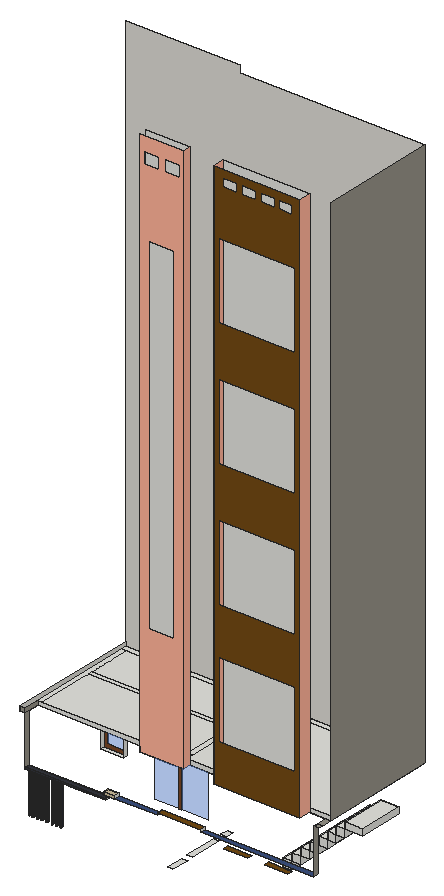
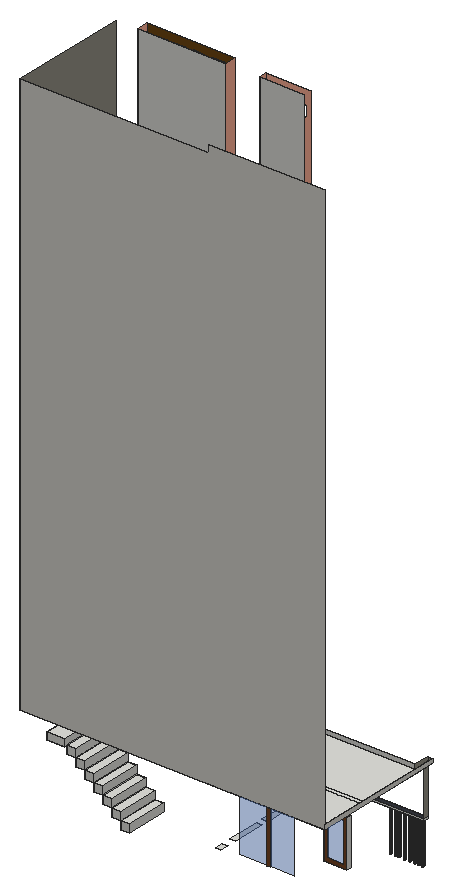
# SketchUp Ruby script. Lengths in inches.
U = 1.inch
M = Sketchup.active_model
def pt(a) = Geom::Point3d.new(a.map { |v| v * U })
def face(e, loops, mat)
  f = e.add_face(loops[0].map { |a| pt(a) })
  loops[1..].each { |l| e.add_face(l.map { |a| pt(a) }).erase! }
  f.material = f.back_material = mat if mat
  f
end
# faces: each face lists its corners as indices into pts; further lists are holes
def faces(e, pts, list, mat = nil) = list.each { |f| face(e, (f[0].is_a?(Array) ? f : [f]).map { |l| l.map { |i| pts[i] } }, mat) }
# xy, xz, yz: faces in a plane at the given z, y or x. An outline is a flat list of corners, or four numbers for a rectangle; further outlines are holes
def ring(l) = l.size == 4 ? [[l[0], l[1]], [l[2], l[1]], [l[2], l[3]], [l[0], l[3]]] : l.each_slice(2).to_a
def flat(e, list, mat, &to3) = list.each { |f| face(e, (f[0].is_a?(Array) ? f : [f]).map { |l| ring(l).map { |u, v| to3.(u, v) } }, mat) }
def xy(e, z, list, mat = nil) = flat(e, list, mat) { |x, y| [x, y, z] }
def xz(e, y, list, mat = nil) = flat(e, list, mat) { |x, z| [x, y, z] }
def yz(e, x, list, mat = nil) = flat(e, list, mat) { |y, z| [x, y, z] }
def lines(e, pts, list) = list.each { |a, b| e.add_line(pt(pts[a]), pt(pts[b])) }
# prism: a flat outline (further loops are holes) pulled along v
def prism(e, loops, v, mat = nil)
  f = face(e, loops, mat); d = Geom::Vector3d.new(v.map { |x| x * U })
  f.pushpull(f.normal.samedirection?(d) ? d.length : -d.length)
end
def box(e, o, s, mat = nil) = prism(e, [[o, [o[0] + s[0], o[1], o[2]], [o[0] + s[0], o[1] + s[1], o[2]], [o[0], o[1] + s[1], o[2]]]], [0, 0, s[2]], mat)
def at(x, y, z, deg = 0) = Geom::Transformation.translation(pt([x, y, z])) * Geom::Transformation.rotation(ORIGIN, Z_AXIS, deg.degrees)
def axes(o, x, y, z) = Geom::Transformation.new([*x, 0, *y, 0, *z, 0, *pt(o).to_a, 1])
def part(name) = M.definitions.add(name)
# library, detail: a bought-in or finely detailed component or shape, given as its bounding box
def library(name, o, s) = part(name).tap { |d| box(d.entities, o, s) }
def detail(e, o, s) = box(e.add_group.entities, o, s)
def put(e, d, t, mat = nil) = e.add_instance(d, t).tap { |i| i.material = mat if mat }
def group(e, t, mat = nil) = e.add_group.tap { |g| g.transformation = t; g.material = mat if mat }.entities
root = M.entities
M.materials.add("[Blinds Weave]").color = [114, 74, 20]
M.materials.add("[Color B02]").color = [255, 178, 153]
M.materials.add("[Formica Blue]").color = [58, 79, 124]
M.materials.add("[Formica Graystone]").color = [149, 146, 135]
M.materials.add("[Formica Laminate Dark]").color = [50, 53, 60]
M.materials.add("[Quartz Light Brown]").color = [199, 184, 152]
M.materials.add("[Terrazzo Tile Light]").color = [219, 217, 210]
M.materials.add("[Translucent Glass Blue]").color = [100, 149, 237]
M.materials["[Translucent Glass Blue]"].alpha = 0.5
M.materials.add("[Wood Veneer 01]").color = [120, 70, 37]
xy(root,9,[[405.97,32.04,421.1,82.09],[405.97,100.35,421.1,192.875],[405.97,220.7,421.1,243]])
xy(root,9.5,[[43.24,22.63,42.52,22.73,41.86,23,41.29,23.4375,40.85,24.01,40.58,24.67,40.49,25.38,40.58,26.09,40.85,26.76,41.29,27.33,41.86,27.76,42.52,28.04,43.24,28.13,43.95,28.04,44.61,27.76,45.18,27.33,45.62,26.76,45.89,26.09,45.99,25.38,45.89,24.67,45.62,24.01,45.18,23.4375,44.61,23,43.95,22.73]])
xy(root,90.32,[[48.09,243,111.9,254.6875]])
xy(root,121.625,[[575.75,18.26,642.4375,31.76],[690.75,18.26,757.4375,31.45]],"[Blinds Weave]")
xy(root,126.29,[[[13.78,18.26,120.72,32.04],[109.61,22.63,110.32,22.73,110.99,23,111.56,23.4375,111.99,24.01,112.27,24.67,112.36,25.38,112.27,26.09,111.99,26.76,111.56,27.33,110.99,27.76,110.32,28.04,109.61,28.13,108.9,28.04,108.24,27.76,107.67,27.33,107.23,26.76,106.95,26.09,106.86,25.38,106.95,24.67,107.23,24.01,107.67,23.4375,108.24,23,108.9,22.73],[96.86,22.63,97.57,22.73,98.24,23,98.81,23.4375,99.24,24.01,99.52,24.67,99.61,25.38,99.52,26.09,99.24,26.76,98.81,27.33,98.24,27.76,97.57,28.04,96.86,28.13,96.15,28.04,95.49,27.76,94.92,27.33,94.48,26.76,94.2,26.09,94.11,25.38,94.2,24.67,94.48,24.01,94.92,23.4375,95.49,23,96.15,22.73],[86.17,22.63,86.89,22.73,87.55,23,88.12,23.4375,88.55,24.01,88.83,24.67,88.92,25.38,88.83,26.09,88.55,26.76,88.12,27.33,87.55,27.76,86.89,28.04,86.17,28.13,85.46,28.04,84.8,27.76,84.23,27.33,83.79,26.76,83.52,26.09,83.42,25.38,83.52,24.67,83.79,24.01,84.23,23.4375,84.8,23,85.46,22.73],[70.8,22.63,71.51,22.73,72.17,23,72.74,23.4375,73.18,24.01,73.45,24.67,73.55,25.38,73.45,26.09,73.18,26.76,72.74,27.33,72.17,27.76,71.51,28.04,70.8,28.13,70.09,28.04,69.42,27.76,68.85,27.33,68.42,26.76,68.14,26.09,68.05,25.38,68.14,24.67,68.42,24.01,68.85,23.4375,69.42,23,70.09,22.73],[56.49,22.63,57.2,22.73,57.86,23,58.43,23.4375,58.87,24.01,59.14,24.67,59.24,25.38,59.14,26.09,58.87,26.76,58.43,27.33,57.86,27.76,57.2,28.04,56.49,28.13,55.77,28.04,55.11,27.76,54.54,27.33,54.1,26.76,53.83,26.09,53.74,25.38,53.83,24.67,54.1,24.01,54.54,23.4375,55.11,23,55.77,22.73],[43.24,22.63,43.95,22.73,44.61,23,45.18,23.4375,45.62,24.01,45.89,24.67,45.99,25.38,45.89,26.09,45.62,26.76,45.18,27.33,44.61,27.76,43.95,28.04,43.24,28.13,42.52,28.04,41.86,27.76,41.29,27.33,40.85,26.76,40.58,26.09,40.49,25.38,40.58,24.67,40.85,24.01,41.29,23.4375,41.86,23,42.52,22.73],[31.74,22.63,32.45,22.73,33.11,23,33.68,23.4375,34.12,24.01,34.39,24.67,34.49,25.38,34.39,26.09,34.12,26.76,33.68,27.33,33.11,27.76,32.45,28.04,31.74,28.13,31.02,28.04,30.36,27.76,29.79,27.33,29.35,26.76,29.08,26.09,28.99,25.38,29.08,24.67,29.35,24.01,29.79,23.4375,30.36,23,31.02,22.73],[20.55,22.63,21.26,22.73,21.92,23,22.49,23.4375,22.93,24.01,23.2,24.67,23.3,25.38,23.2,26.09,22.93,26.76,22.49,27.33,21.92,27.76,21.26,28.04,20.55,28.13,19.84,28.04,19.17,27.76,18.6,27.33,18.17,26.76,17.89,26.09,17.8,25.38,17.89,24.67,18.17,24.01,18.6,23.4375,19.17,23,19.84,22.73]],[131.16,18.26,141.6,32.04],[[141.6,18.26,240.76,32.04],[229.92,22.63,230.64,22.73,231.3,23,231.87,23.4375,232.3,24.01,232.58,24.67,232.67,25.38,232.58,26.09,232.3,26.76,231.87,27.33,231.3,27.76,230.64,28.04,229.92,28.13,229.21,28.04,228.55,27.76,227.98,27.33,227.54,26.76,227.27,26.09,227.17,25.38,227.27,24.67,227.54,24.01,227.98,23.4375,228.55,23,229.21,22.73],[218.67,22.63,219.39,22.73,220.05,23,220.62,23.4375,221.05,24.01,221.33,24.67,221.42,25.38,221.33,26.09,221.05,26.76,220.62,27.33,220.05,27.76,219.39,28.04,218.67,28.13,217.96,28.04,217.3,27.76,216.73,27.33,216.29,26.76,216.02,26.09,215.92,25.38,216.02,24.67,216.29,24.01,216.73,23.4375,217.3,23,217.96,22.73],[209.17,22.63,209.89,22.73,210.55,23,211.12,23.4375,211.55,24.01,211.83,24.67,211.92,25.38,211.83,26.09,211.55,26.76,211.12,27.33,210.55,27.76,209.89,28.04,209.17,28.13,208.46,28.04,207.8,27.76,207.23,27.33,206.79,26.76,206.52,26.09,206.42,25.38,206.52,24.67,206.79,24.01,207.23,23.4375,207.8,23,208.46,22.73],[197.05,22.63,197.76,22.73,198.42,23,198.99,23.4375,199.43,24.01,199.7,24.67,199.8,25.38,199.7,26.09,199.43,26.76,198.99,27.33,198.42,27.76,197.76,28.04,197.05,28.13,196.34,28.04,195.67,27.76,195.1,27.33,194.67,26.76,194.39,26.09,194.3,25.38,194.39,24.67,194.67,24.01,195.1,23.4375,195.67,23,196.34,22.73],[183.8,22.63,184.51,22.73,185.17,23,185.74,23.4375,186.18,24.01,186.45,24.67,186.55,25.38,186.45,26.09,186.18,26.76,185.74,27.33,185.17,27.76,184.51,28.04,183.8,28.13,183.09,28.04,182.42,27.76,181.85,27.33,181.42,26.76,181.14,26.09,181.05,25.38,181.14,24.67,181.42,24.01,181.85,23.4375,182.42,23,183.09,22.73],[171.74,22.63,172.45,22.73,173.11,23,173.68,23.4375,174.12,24.01,174.39,24.67,174.49,25.38,174.39,26.09,174.12,26.76,173.68,27.33,173.11,27.76,172.45,28.04,171.74,28.13,171.02,28.04,170.36,27.76,169.79,27.33,169.35,26.76,169.08,26.09,168.99,25.38,169.08,24.67,169.35,24.01,169.79,23.4375,170.36,23,171.02,22.73],[160.92,22.63,161.64,22.73,162.3,23,162.87,23.4375,163.3,24.01,163.58,24.67,163.67,25.38,163.58,26.09,163.3,26.76,162.87,27.33,162.3,27.76,161.64,28.04,160.92,28.13,160.21,28.04,159.55,27.76,158.98,27.33,158.54,26.76,158.27,26.09,158.17,25.38,158.27,24.67,158.54,24.01,158.98,23.4375,159.55,23,160.21,22.73],[150.24,22.63,150.95,22.73,151.61,23,152.18,23.4375,152.62,24.01,152.89,24.67,152.99,25.38,152.89,26.09,152.62,26.76,152.18,27.33,151.61,27.76,150.95,28.04,150.24,28.13,149.52,28.04,148.86,27.76,148.29,27.33,147.85,26.76,147.58,26.09,147.49,25.38,147.58,24.67,147.85,24.01,148.29,23.4375,148.86,23,149.52,22.73]]])
xy(root,130.36,[[13.78,18.26,240.76,32.04]],"[Formica Laminate Dark]")
xy(root,140.3125,[[237.58,15.64,265.93,18.26],[265.93,15.64,268.05,18.26],[237.58,18.26,240.76,32.04],[240.76,18.26,265.93,32.04],[265.93,18.26,268.05,32.04]])
xy(root,140.3125,[[268.05,18.26,388.35,32.04],[510.77,18.26,829.54,32.04]],"[Formica Blue]")
xy(root,146.9375,[[388.35,18.26,510.77,32.04]],"[Blinds Weave]")
xy(root,147.25,[[237.58,15.64,268.05,32.04]],"[Quartz Light Brown]")
xy(root,219.95,[[48.09,243,111.9,254.6875]])
xy(root,267.75,[[0,18.26,13.78,32.04],[538.37,28.0625,782.27,61.625],[0,32.04,13.78,377.76],[320.63,40.625,405.97,61.625],[405.97,40.625,421.1,61.625],
  [421.1,40.625,443.82,61.625],[13.78,61.625,405.97,243],[405.97,61.625,421.1,82.09],[421.1,61.625,829.54,377.76],[829.54,61.625,843.32,377.76],
  [405.97,82.09,421.1,100.35],[405.97,100.35,421.1,192.875],[405.97,192.875,421.1,220.7],[405.97,220.7,421.1,243],[13.78,243,405.97,255.17],
  [405.97,243,421.1,391.54],[13.78,255.17,405.97,377.76],[0,377.76,405.97,391.54],[421.1,377.76,843.32,391.54]])
xy(root,267.75,[[829.54,18.26,843.32,32.04],[829.54,32.04,843.32,61.625]],"[Formica Graystone]")
xz(root,15.64,[[237.58,140.3125,268.05,147.25]],"[Quartz Light Brown]")
xz(root,18.26,[[0,267.75,13.78,279.75]],"[Formica Graystone]")
xz(root,18.26,[[13.78,126.29,240.76,130.36]],"[Formica Laminate Dark]")
xz(root,28.0625,[[[538.37,267.75,782.27,1831.875],[552.31,378.36,767.87,593.92],[552.31,726.11,767.87,941.67],[552.31,1082.8,767.87,1298.36],[552.31,1440.48,767.87,1656.05],[565.47,1787.53,604,1811.34],[721.9,1787.53,760.43,1811.34],[618.59,1787.53,657.12,1811.34],[671.78,1787.53,710.31,1811.34]]],"[Blinds Weave]")
xz(root,32.04,[[13.78,126.29,240.76,130.36],[237.58,140.3125,268.05,147.25]])
xz(root,40.625,[[[320.63,267.75,443.82,1831.875],[345.55,586.3125,414.87,1568.875],[331.73,1759.52,372.85,1792.7],[390.85,1759.52,431.98,1792.7]]],"[Color B02]")
xz(root,61.625,[[13.78,267.75,320.63,279.75],[320.63,267.75,443.82,1831.875],[443.82,267.75,538.37,280.75],[538.37,267.75,782.27,1831.875],[782.27,267.75,843.32,278.91]])
xz(root,243,[[200.58,15.66,268.66,218.84],[278.13,15.66,352.51,218.84]],"[Translucent Glass Blue]")
xz(root,243,[[268.66,15.66,278.13,218.84]],"[Wood Veneer 01]")
xz(root,254.6875,[[57.74,99.98,102.25,210.29]],"[Translucent Glass Blue]")
xz(root,254.6875,[[[48.09,90.32,111.9,219.95],[57.74,99.98,102.25,210.29]]],"[Wood Veneer 01]")
xz(root,391.54,[[0,267.75,0,1852.125,320.63,1852.125,320.63,1831.875,843.32,1831.875,843.32,267.75]],"[Terrazzo Tile Light]")
yz(root,0,[[18.26,267.75,391.54,279.75]],"[Terrazzo Tile Light]")
yz(root,13.78,[[18.26,126.29,32.04,130.36]])
yz(root,13.78,[[18.26,130.36,32.04,267.75],[18.26,267.75,61.625,279.75]],"[Formica Graystone]")
yz(root,48.09,[[243,90.32,254.6875,219.95]])
yz(root,111.9,[[243,90.32,254.6875,219.95]])
yz(root,237.58,[[15.64,140.3125,32.04,147.25]],"[Quartz Light Brown]")
yz(root,240.76,[[18.26,126.29,32.04,130.36]])
yz(root,240.76,[[18.26,130.36,32.04,140.3125]],"[Quartz Light Brown]")
yz(root,268.05,[[15.64,140.3125,32.04,147.25]])
yz(root,320.63,[[40.625,267.75,61.625,279.75]])
yz(root,388.35,[[18.26,140.3125,32.04,146.9375]])
yz(root,443.82,[[40.625,267.75,61.625,1831.875]],"[Color B02]")
yz(root,510.77,[[18.26,140.3125,32.04,146.9375]])
yz(root,538.37,[[28.0625,267.75,61.625,1831.875]],"[Color B02]")
yz(root,782.27,[[28.0625,267.75,61.625,1831.875]],"[Color B02]")
yz(root,829.54,[[18.26,140.3125,32.04,267.75]],"[Formica Graystone]")
yz(root,843.32,[[61.625,267.75,391.54,1831.875]],"[Formica Graystone]")
p = [[19.84,22.73,9],[20.55,22.63,9],[20.55,22.63,126.29],[19.84,22.73,126.29],[21.26,22.73,9],[21.26,22.73,126.29],
  [31.02,22.73,9],[31.74,22.63,9],[31.74,22.63,126.29],[31.02,22.73,126.29],[32.45,22.73,9],[32.45,22.73,126.29],
  [42.52,22.73,9],[43.24,22.63,9],[43.24,22.63,9.5],[42.52,22.73,9.5],[43.95,22.73,9],[43.95,22.73,9.5],
  [55.77,22.73,9],[56.49,22.63,9],[56.49,22.63,126.29],[55.77,22.73,126.29],[57.2,22.73,9],[57.2,22.73,126.29],
  [70.09,22.73,9],[70.8,22.63,9],[70.8,22.63,126.29],[70.09,22.73,126.29],[71.51,22.73,9],[71.51,22.73,126.29],
  [85.46,22.73,9],[86.17,22.63,9],[86.17,22.63,126.29],[85.46,22.73,126.29],[86.89,22.73,9],[86.89,22.73,126.29],
  [96.15,22.73,9],[96.86,22.63,9],[96.86,22.63,126.29],[96.15,22.73,126.29],[97.57,22.73,9],[97.57,22.73,126.29],
  [19.17,23,9],[19.17,23,126.29],[21.92,23,9],[21.92,23,126.29],[30.36,23,9],[30.36,23,126.29],
  [33.11,23,9],[33.11,23,126.29],[41.86,23,9],[41.86,23,9.5],[44.61,23,9],[44.61,23,9.5],
  [55.11,23,9],[55.11,23,126.29],[57.86,23,9],[57.86,23,126.29],[69.42,23,9],[69.42,23,126.29],
  [72.17,23,9],[72.17,23,126.29],[84.8,23,9],[84.8,23,126.29],[87.55,23,9],[87.55,23,126.29],
  [95.49,23,9],[95.49,23,126.29],[98.24,23,9],[98.24,23,126.29],[18.6,23.4375,9],[18.6,23.4375,126.29],
  [22.49,23.4375,9],[22.49,23.4375,126.29],[29.79,23.4375,9],[29.79,23.4375,126.29],[33.68,23.4375,9],[33.68,23.4375,126.29],
  [41.29,23.4375,9],[41.29,23.4375,9.5],[45.18,23.4375,9],[45.18,23.4375,9.5],[54.54,23.4375,9],[54.54,23.4375,126.29],
  [58.43,23.4375,9],[58.43,23.4375,126.29],[68.85,23.4375,9],[68.85,23.4375,126.29],[72.74,23.4375,9],[72.74,23.4375,126.29],
  [84.23,23.4375,9],[84.23,23.4375,126.29],[88.12,23.4375,9],[88.12,23.4375,126.29],[94.92,23.4375,9],[94.92,23.4375,126.29],
  [98.81,23.4375,9],[98.81,23.4375,126.29],[107.67,23.4375,9],[108.24,23,9],[108.24,23,126.29],[107.67,23.4375,126.29],
  [18.17,24.01,9],[18.17,24.01,126.29],[22.93,24.01,9],[22.93,24.01,126.29],[29.35,24.01,9],[29.35,24.01,126.29],
  [34.12,24.01,9],[34.12,24.01,126.29],[40.85,24.01,9],[40.85,24.01,9.5],[45.62,24.01,9],[45.62,24.01,9.5],
  [54.1,24.01,9],[54.1,24.01,126.29],[58.87,24.01,9],[58.87,24.01,126.29],[68.42,24.01,9],[68.42,24.01,126.29],
  [73.18,24.01,9],[73.18,24.01,126.29],[83.79,24.01,9],[83.79,24.01,126.29],[88.55,24.01,9],[88.55,24.01,126.29],
  [94.48,24.01,9],[94.48,24.01,126.29],[99.24,24.01,9],[99.24,24.01,126.29],[107.23,24.01,9],[107.23,24.01,126.29],
  [111.56,23.4375,9],[111.99,24.01,9],[111.99,24.01,126.29],[111.56,23.4375,126.29],[17.89,24.67,9],[17.89,24.67,126.29],
  [23.2,24.67,9],[23.2,24.67,126.29],[29.08,24.67,9],[29.08,24.67,126.29],[34.39,24.67,9],[34.39,24.67,126.29],
  [40.58,24.67,9],[40.58,24.67,9.5],[45.89,24.67,9],[45.89,24.67,9.5],[53.83,24.67,9],[53.83,24.67,126.29],
  [59.14,24.67,9],[59.14,24.67,126.29],[68.14,24.67,9],[68.14,24.67,126.29],[73.45,24.67,9],[73.45,24.67,126.29],
  [83.52,24.67,9],[83.52,24.67,126.29],[88.83,24.67,9],[88.83,24.67,126.29],[94.2,24.67,9],[94.2,24.67,126.29],
  [99.52,24.67,9],[99.52,24.67,126.29],[106.95,24.67,9],[106.95,24.67,126.29],[112.27,24.67,9],[112.27,24.67,126.29],
  [17.8,25.38,9],[17.8,25.38,126.29],[23.3,25.38,9],[23.3,25.38,126.29],[28.99,25.38,9],[28.99,25.38,126.29],
  [34.49,25.38,9],[34.49,25.38,126.29],[40.49,25.38,9],[40.49,25.38,9.5],[45.99,25.38,9],[45.99,25.38,9.5],
  [53.74,25.38,9],[53.74,25.38,126.29],[59.24,25.38,9],[59.24,25.38,126.29],[68.05,25.38,9],[68.05,25.38,126.29],
  [73.55,25.38,9],[73.55,25.38,126.29],[83.42,25.38,9],[83.42,25.38,126.29],[88.92,25.38,9],[88.92,25.38,126.29],
  [94.11,25.38,9],[94.11,25.38,126.29],[99.61,25.38,9],[99.61,25.38,126.29],[106.86,25.38,9],[106.86,25.38,126.29],
  [112.36,25.38,9],[112.36,25.38,126.29],[17.89,26.09,9],[17.89,26.09,126.29],[23.2,26.09,9],[23.2,26.09,126.29],
  [29.08,26.09,9],[29.08,26.09,126.29],[34.39,26.09,9],[34.39,26.09,126.29],[40.58,26.09,9],[40.58,26.09,9.5],
  [45.89,26.09,9],[45.89,26.09,9.5],[53.83,26.09,9],[53.83,26.09,126.29],[59.14,26.09,9],[59.14,26.09,126.29],
  [68.14,26.09,9],[68.14,26.09,126.29],[73.45,26.09,9],[73.45,26.09,126.29],[83.52,26.09,9],[83.52,26.09,126.29],
  [88.83,26.09,9],[88.83,26.09,126.29],[94.2,26.09,9],[94.2,26.09,126.29],[99.52,26.09,9],[99.52,26.09,126.29],
  [106.95,26.09,9],[106.95,26.09,126.29],[112.27,26.09,9],[112.27,26.09,126.29],[18.17,26.76,9],[18.17,26.76,126.29],
  [22.93,26.76,9],[22.93,26.76,126.29],[29.35,26.76,9],[29.35,26.76,126.29],[34.12,26.76,9],[34.12,26.76,126.29],
  [40.85,26.76,9],[40.85,26.76,9.5],[45.62,26.76,9],[45.62,26.76,9.5],[54.1,26.76,9],[54.1,26.76,126.29],
  [58.87,26.76,9],[58.87,26.76,126.29],[68.42,26.76,9],[68.42,26.76,126.29],[73.18,26.76,9],[73.18,26.76,126.29],
  [83.79,26.76,9],[83.79,26.76,126.29],[88.55,26.76,9],[88.55,26.76,126.29],[94.48,26.76,9],[94.48,26.76,126.29],
  [99.24,26.76,9],[99.24,26.76,126.29],[107.23,26.76,9],[107.23,26.76,126.29],[111.99,26.76,9],[111.99,26.76,126.29],
  [18.6,27.33,9],[18.6,27.33,126.29],[22.49,27.33,9],[22.49,27.33,126.29],[29.79,27.33,9],[29.79,27.33,126.29],
  [33.68,27.33,9],[33.68,27.33,126.29],[41.29,27.33,9],[41.29,27.33,9.5],[45.18,27.33,9],[45.18,27.33,9.5],
  [54.54,27.33,9],[54.54,27.33,126.29],[58.43,27.33,9],[58.43,27.33,126.29],[68.85,27.33,9],[68.85,27.33,126.29],
  [72.74,27.33,9],[72.74,27.33,126.29],[84.23,27.33,9],[84.23,27.33,126.29],[88.12,27.33,9],[88.12,27.33,126.29],
  [94.92,27.33,9],[94.92,27.33,126.29],[98.81,27.33,9],[98.81,27.33,126.29],[107.67,27.33,9],[107.67,27.33,126.29],
  [111.56,27.33,9],[111.56,27.33,126.29],[19.17,27.76,9],[19.17,27.76,126.29],[21.92,27.76,9],[21.92,27.76,126.29],
  [30.36,27.76,9],[30.36,27.76,126.29],[33.11,27.76,9],[33.11,27.76,126.29],[41.86,27.76,9],[41.86,27.76,9.5],
  [44.61,27.76,9],[44.61,27.76,9.5],[55.11,27.76,9],[55.11,27.76,126.29],[57.86,27.76,9],[57.86,27.76,126.29],
  [69.42,27.76,9],[69.42,27.76,126.29],[72.17,27.76,9],[72.17,27.76,126.29],[84.8,27.76,9],[84.8,27.76,126.29],
  [87.55,27.76,9],[87.55,27.76,126.29],[95.49,27.76,9],[95.49,27.76,126.29],[98.24,27.76,9],[98.24,27.76,126.29],
  [108.24,27.76,9],[108.24,27.76,126.29],[110.99,27.76,9],[110.99,27.76,126.29],[19.84,28.04,9],[19.84,28.04,126.29],
  [21.26,28.04,9],[21.26,28.04,126.29],[31.02,28.04,9],[31.02,28.04,126.29],[32.45,28.04,9],[32.45,28.04,126.29],
  [42.52,28.04,9],[42.52,28.04,9.5],[43.95,28.04,9],[43.95,28.04,9.5],[55.77,28.04,9],[55.77,28.04,126.29],
  [57.2,28.04,9],[57.2,28.04,126.29],[70.09,28.04,9],[70.09,28.04,126.29],[71.51,28.04,9],[71.51,28.04,126.29],
  [85.46,28.04,9],[85.46,28.04,126.29],[86.89,28.04,9],[86.89,28.04,126.29],[96.15,28.04,9],[96.15,28.04,126.29],
  [97.57,28.04,9],[97.57,28.04,126.29],[108.9,28.04,9],[108.9,28.04,126.29],[110.32,28.04,9],[110.32,28.04,126.29],
  [20.55,28.13,9],[20.55,28.13,126.29],[31.74,28.13,9],[31.74,28.13,126.29],[43.24,28.13,9],[43.24,28.13,9.5],
  [56.49,28.13,9],[56.49,28.13,126.29],[70.8,28.13,9],[70.8,28.13,126.29],[86.17,28.13,9],[86.17,28.13,126.29],
  [96.86,28.13,9],[96.86,28.13,126.29],[109.61,28.13,9],[109.61,28.13,126.29],[43.24,22.63,126.29],[42.52,22.73,126.29],
  [43.95,22.73,126.29],[41.86,23,126.29],[44.61,23,126.29],[41.29,23.4375,126.29],[45.18,23.4375,126.29],[40.85,24.01,126.29],
  [45.62,24.01,126.29],[40.58,24.67,126.29],[45.89,24.67,126.29],[40.49,25.38,126.29],[45.99,25.38,126.29],[40.58,26.09,126.29],
  [45.89,26.09,126.29],[40.85,26.76,126.29],[45.62,26.76,126.29],[41.29,27.33,126.29],[45.18,27.33,126.29],[41.86,27.76,126.29],
  [44.61,27.76,126.29],[42.52,28.04,126.29],[43.95,28.04,126.29],[43.24,28.13,126.29]]
faces(root,p,[[0,1,2,3],[1,4,5,2],[6,7,8,9],[7,10,11,8],[18,19,20,21],[19,22,23,20],[24,25,26,27],[25,28,29,26],
  [30,31,32,33],[31,34,35,32],[36,37,38,39],[37,40,41,38],[42,0,3,43],[4,44,45,5],[46,6,9,47],[10,48,49,11],
  [54,18,21,55],[22,56,57,23],[58,24,27,59],[28,60,61,29],[62,30,33,63],[34,64,65,35],[66,36,39,67],[40,68,69,41],
  [70,42,43,71],[44,72,73,45],[74,46,47,75],[48,76,77,49],[82,54,55,83],[56,84,85,57],[86,58,59,87],[60,88,89,61],
  [90,62,63,91],[64,92,93,65],[94,66,67,95],[68,96,97,69],[98,99,100,101],[102,70,71,103],[72,104,105,73],[106,74,75,107],
  [76,108,109,77],[114,82,83,115],[84,116,117,85],[118,86,87,119],[88,120,121,89],[122,90,91,123],[92,124,125,93],[126,94,95,127],
  [96,128,129,97],[130,98,101,131],[132,133,134,135],[136,102,103,137],[104,138,139,105],[140,106,107,141],[108,142,143,109],[148,114,115,149],
  [116,150,151,117],[152,118,119,153],[120,154,155,121],[156,122,123,157],[124,158,159,125],[160,126,127,161],[128,162,163,129],[164,130,131,165],
  [133,166,167,134],[168,136,137,169],[138,170,171,139],[172,140,141,173],[142,174,175,143],[180,148,149,181],[150,182,183,151],[184,152,153,185],
  [154,186,187,155],[188,156,157,189],[158,190,191,159],[192,160,161,193],[162,194,195,163],[196,164,165,197],[166,198,199,167],[200,168,169,201],
  [170,202,203,171],[204,172,173,205],[174,206,207,175],[212,180,181,213],[182,214,215,183],[216,184,185,217],[186,218,219,187],[220,188,189,221],
  [190,222,223,191],[224,192,193,225],[194,226,227,195],[228,196,197,229],[198,230,231,199],[232,200,201,233],[202,234,235,203],[236,204,205,237],
  [206,238,239,207],[244,212,213,245],[214,246,247,215],[248,216,217,249],[218,250,251,219],[252,220,221,253],[222,254,255,223],[256,224,225,257],
  [226,258,259,227],[260,228,229,261],[230,262,263,231],[264,232,233,265],[234,266,267,235],[268,236,237,269],[238,270,271,239],[276,244,245,277],
  [246,278,279,247],[280,248,249,281],[250,282,283,251],[284,252,253,285],[254,286,287,255],[288,256,257,289],[258,290,291,259],[292,260,261,293],
  [262,294,295,263],[296,264,265,297],[266,298,299,267],[300,268,269,301],[270,302,303,271],[308,276,277,309],[278,310,311,279],[312,280,281,313],
  [282,314,315,283],[316,284,285,317],[286,318,319,287],[320,288,289,321],[290,322,323,291],[324,292,293,325],[294,326,327,295],[328,296,297,329],
  [298,330,331,299],[332,300,301,333],[302,334,335,303],[340,308,309,341],[310,342,343,311],[344,312,313,345],[314,346,347,315],[348,316,317,349],
  [318,350,351,319],[352,320,321,353],[322,354,355,323],[356,324,325,357],[326,358,359,327],[360,328,329,361],[330,360,361,331],[362,332,333,363],
  [334,362,363,335],[366,340,341,367],[342,366,367,343],[368,344,345,369],[346,368,369,347],[370,348,349,371],[350,370,371,351],[372,352,353,373],
  [354,372,373,355],[374,356,357,375],[358,374,375,359],[15,14,376,377],[14,17,378,376],[51,15,377,379],[17,53,380,378],[79,51,379,381],
  [53,81,382,380],[111,79,381,383],[81,113,384,382],[145,111,383,385],[113,147,386,384],[177,145,385,387],[147,179,388,386],[209,177,387,389],
  [179,211,390,388],[241,209,389,391],[211,243,392,390],[273,241,391,393],[243,275,394,392],[305,273,393,395],[275,307,396,394],[337,305,395,397],
  [307,339,398,396],[365,337,397,399],[339,365,399,398]],"[Formica Laminate Dark]")
faces(root,p,[[12,13,14,15],[13,16,17,14],[50,12,15,51],[16,52,53,17],[78,50,51,79],[52,80,81,53],[110,78,79,111],[80,112,113,81],
  [144,110,111,145],[112,146,147,113],[176,144,145,177],[146,178,179,147],[208,176,177,209],[178,210,211,179],[240,208,209,241],[210,242,243,211],
  [272,240,241,273],[242,274,275,243],[304,272,273,305],[274,306,307,275],[336,304,305,337],[306,338,339,307],[364,336,337,365],[338,364,365,339]])
g1 = group(root,at(605,190.91,10.36))
xy(g1,0,[[0,0,24.97,118.43]])
xy(g1,22.35,[[0,0,24.97,118.43],[24.97,0,49.93,118.43]])
xy(g1,44.71,[[24.97,0,49.93,118.43],[49.93,0,74.9,118.43]])
xy(g1,67.0625,[[49.93,0,74.9,118.43],[74.9,0,99.87,118.43]])
xy(g1,89.42,[[74.9,0,99.87,118.43],[99.87,0,124.83,118.43]])
xy(g1,111.77,[[99.87,0,124.83,118.43],[124.83,0,149.8,118.43]])
xy(g1,134.125,[[124.83,0,149.8,118.43],[149.8,0,174.77,118.43]])
xy(g1,156.48,[[149.8,0,174.77,118.43],[174.77,0,224.54,126.5]])
xy(g1,174.91,[[174.77,0,224.54,126.5]])
xz(g1,0,[[0,0,24.97,22.35],[24.97,22.35,49.93,44.71],[49.93,44.71,74.9,67.0625],[74.9,67.0625,99.87,89.42],[99.87,89.42,124.83,111.77],
  [124.83,111.77,149.8,134.125],[149.8,134.125,174.77,156.48],[174.77,156.48,224.54,174.91]])
xz(g1,118.43,[[0,0,24.97,22.35],[24.97,22.35,49.93,44.71],[49.93,44.71,74.9,67.0625],[74.9,67.0625,99.87,89.42],[99.87,89.42,124.83,111.77],
  [124.83,111.77,149.8,134.125],[149.8,134.125,174.77,156.48]])
xz(g1,126.5,[[174.77,156.48,224.54,174.91]])
yz(g1,0,[[0,0,118.43,22.35]])
yz(g1,24.97,[[0,0,118.43,22.35],[0,22.35,118.43,44.71]])
yz(g1,49.93,[[0,22.35,118.43,44.71],[0,44.71,118.43,67.0625]])
yz(g1,74.9,[[0,44.71,118.43,67.0625],[0,67.0625,118.43,89.42]])
yz(g1,99.87,[[0,67.0625,118.43,89.42],[0,89.42,118.43,111.77]])
yz(g1,124.83,[[0,89.42,118.43,111.77],[0,111.77,118.43,134.125]])
yz(g1,149.8,[[0,111.77,118.43,134.125],[0,134.125,118.43,156.48]])
yz(g1,174.77,[[0,134.125,118.43,156.48],[0,156.48,126.5,174.91]])
yz(g1,224.54,[[0,156.48,126.5,174.91]])
